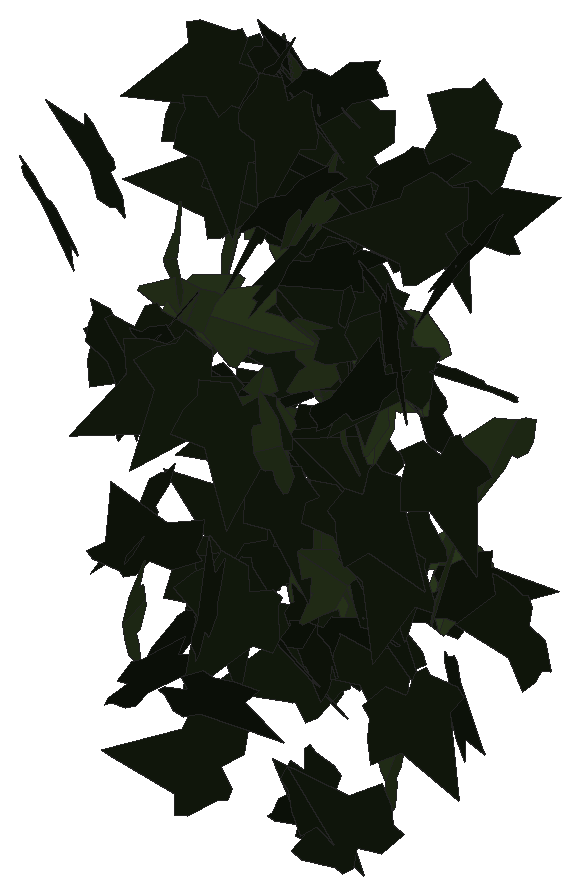
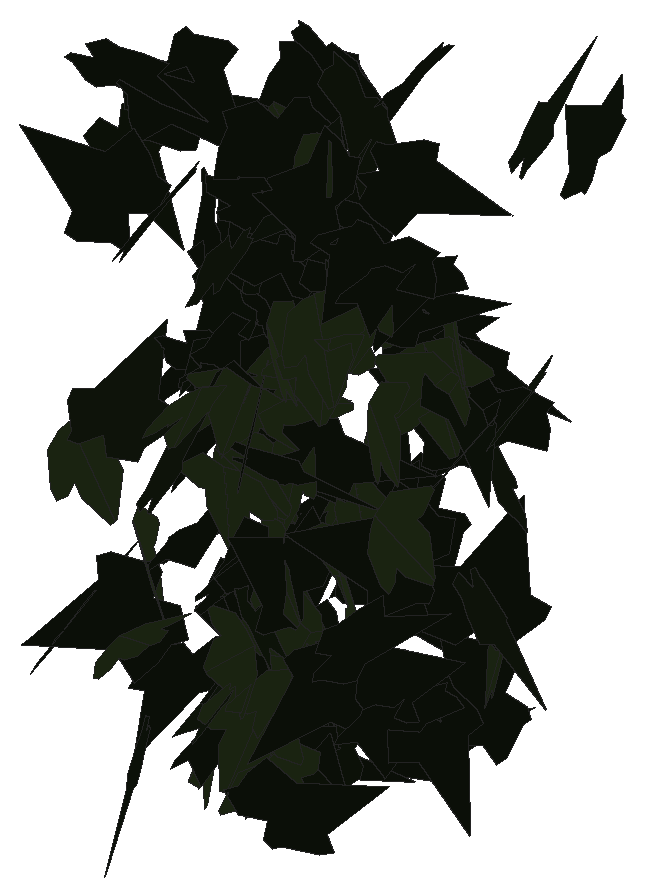
# SketchUp Ruby script. Lengths in inches.
U = 1.inch
M = Sketchup.active_model
def pt(a) = Geom::Point3d.new(a.map { |v| v * U })
def face(e, loops, mat)
  f = e.add_face(loops[0].map { |a| pt(a) })
  loops[1..].each { |l| e.add_face(l.map { |a| pt(a) }).erase! }
  f.material = f.back_material = mat if mat
  f
end
# faces: each face lists its corners as indices into pts; further lists are holes
def faces(e, pts, list, mat = nil) = list.each { |f| face(e, (f[0].is_a?(Array) ? f : [f]).map { |l| l.map { |i| pts[i] } }, mat) }
# xy, xz, yz: faces in a plane at the given z, y or x. An outline is a flat list of corners, or four numbers for a rectangle; further outlines are holes
def ring(l) = l.size == 4 ? [[l[0], l[1]], [l[2], l[1]], [l[2], l[3]], [l[0], l[3]]] : l.each_slice(2).to_a
def flat(e, list, mat, &to3) = list.each { |f| face(e, (f[0].is_a?(Array) ? f : [f]).map { |l| ring(l).map { |u, v| to3.(u, v) } }, mat) }
def xy(e, z, list, mat = nil) = flat(e, list, mat) { |x, y| [x, y, z] }
def xz(e, y, list, mat = nil) = flat(e, list, mat) { |x, z| [x, y, z] }
def yz(e, x, list, mat = nil) = flat(e, list, mat) { |y, z| [x, y, z] }
def lines(e, pts, list) = list.each { |a, b| e.add_line(pt(pts[a]), pt(pts[b])) }
# prism: a flat outline (further loops are holes) pulled along v
def prism(e, loops, v, mat = nil)
  f = face(e, loops, mat); d = Geom::Vector3d.new(v.map { |x| x * U })
  f.pushpull(f.normal.samedirection?(d) ? d.length : -d.length)
end
def box(e, o, s, mat = nil) = prism(e, [[o, [o[0] + s[0], o[1], o[2]], [o[0] + s[0], o[1] + s[1], o[2]], [o[0], o[1] + s[1], o[2]]]], [0, 0, s[2]], mat)
def at(x, y, z, deg = 0) = Geom::Transformation.translation(pt([x, y, z])) * Geom::Transformation.rotation(ORIGIN, Z_AXIS, deg.degrees)
def axes(o, x, y, z) = Geom::Transformation.new([*x, 0, *y, 0, *z, 0, *pt(o).to_a, 1])
def part(name) = M.definitions.add(name)
# library, detail: a bought-in or finely detailed component or shape, given as its bounding box
def library(name, o, s) = part(name).tap { |d| box(d.entities, o, s) }
def detail(e, o, s) = box(e.add_group.entities, o, s)
def put(e, d, t, mat = nil) = e.add_instance(d, t).tap { |i| i.material = mat if mat }
def group(e, t, mat = nil) = e.add_group.tap { |g| g.transformation = t; g.material = mat if mat }.entities
root = M.entities
M.materials.add("efeu1").color = [18, 25, 13]
M.materials.add("efeu2").color = [43, 57, 29]
c1 = part("ivyleaf_9")
p = [[1.54,2.16,1.25],[1.36,2.04,1.19],[-0.21,0.99,0.68],[-0.71,1.11,0.82],[-0.85,0.86,0.67],[-0.8,0.17,0.21],
  [-0.9,-0.01,0.1],[-0.67,-0.16,-0.02],[-0.08,-0.08,-0.05],[-0.03,-0.6,-0.4],[0.65,-0.88,-0.66],[0.83,-0.6,-0.49],
  [1.29,-0.42,-0.43],[1.8125,-0.07,-0.26],[1.21,0.44,0.15]]
faces(c1.entities,p,[[0,1,2,3,4,5,6,7,8,9,10,11,12,13,14]],"efeu1")
c2 = part("ivyleaf_10")
p = [[0,0.5,-0.03],[-0.0625,2.02,-0.43],[-0.19,2.01,-0.46],[-0.54,1.05,-0.29],[-0.52,0.625,-0.18],[-0.83,0.76,-0.28],
  [-1.16,0.64,-0.33],[-1.15,0.33,-0.24],[-0.77,-0.39,0.02],[-0.3,-0.51,0.16],[0.04,-0.48,0.23],[-0.02,2.01,-0.4375],
  [-0.06,2.01,-0.43],[0.04,-0.49,0.23],[0.67,-0.49,0.14],[1.38,0.36,-0.2],[1.375,0.51,-0.24],[0.81,0.65,-0.19],
  [0.62,0.59,-0.15],[0.6,1.09,-0.28],[0.5,1.23,-0.31]]
faces(c2.entities,p,[[0,1,2,3,4,5,6,7,8,9,10],[11,12,0,13,14,15,16,17,18,19,20]],"efeu2")
put(root,c1,axes([47.28,216.89,235.39],[0.45431,0.18289,0.10075],[0.09275,0.0394,-0.48974],[-0.18708,0.46368,0.00187]))
put(root,c1,axes([44.5625,217.46,241],[0.14292,-0.31641,0.35981],[0.16736,-0.31886,-0.34687],[0.44896,0.21958,0.01477]))
put(root,c1,axes([49.17,217.66,233.6],[0.12864,0.03086,0.48218],[-0.4817,0.0471,0.12549],[-0.03767,-0.49682,0.04185]))
put(root,c1,axes([48.48,217.62,234.32],[0.29957,-0.33555,-0.21831],[-0.12796,0.17811,-0.44934],[0.37932,0.32509,0.02084]))
put(root,c1,axes([47.18,217.97,238.78],[-0.20004,-0.4453,-0.10814],[0.0408,0.10022,-0.48815],[0.45642,-0.20412,-0.00376]))
put(root,c2,axes([47.98,217.66,238.68],[-0.22897,0.0956,0.43409],[-0.43182,0.06792,-0.24273],[-0.10538,-0.48605,0.05146]))
put(root,c1,axes([48.26,217.8125,233.48],[0.39361,0.26764,-0.15311],[0.12772,0.08446,0.47598],[0.28064,-0.41381,-0.00188]))
put(root,c1,axes([44.93,218.18,241.22],[0.19498,-0.45249,0.08506],[-0.02724,0.08087,0.49266],[-0.45961,-0.19675,0.00689]))
put(root,c1,axes([46.44,218.41,233.39],[-0.1512,-0.06618,0.47197],[-0.43354,-0.18655,-0.16504],[0.19794,-0.45915,-0.00097]))
put(root,c1,axes([45.84,218.32,238.45],[-0.46631,-0.01893,0.17942],[-0.17944,-0.00299,-0.46668],[0.01874,-0.49963,-0.004]))
put(root,c1,axes([46.72,217.84,235.67],[-0.01158,0.13161,0.48223],[-0.0926,0.47344,-0.13144],[-0.49121,-0.09236,0.01341]))
put(root,c1,axes([46.23,218.48,238.66],[-0.36119,-0.32993,0.10337],[-0.0728,-0.07356,-0.48917],[0.33799,-0.36842,0.0051]))
put(root,c1,axes([45.38,218.1,234.3125],[0.24314,0.25187,0.35699],[0.1949,0.30312,-0.3466],[-0.39102,0.3077,0.04922]))
put(root,c2,axes([45.29,218.2,235.1],[-0.03687,0.11331,0.4856],[-0.32453,0.36423,-0.10963],[-0.37858,-0.32326,0.04669]))
put(root,c1,axes([46.55,218.84,235.6],[-0.43672,-0.23988,-0.04162],[0.04043,0.01284,-0.4982],[0.24008,-0.43851,0.00818]))
put(root,c1,axes([48.26,218.67,238.86],[0.26417,0.36513,0.21655],[-0.12708,-0.17534,0.45067],[0.40505,-0.29314,0.00017]))
put(root,c1,axes([45.07,218.82,235.625],[0.34526,0.08136,0.35238],[-0.34374,-0.07758,0.35471],[0.1124,-0.4872,0.00236]))
put(root,c1,axes([46.08,218.91,241.97],[0.08588,-0.49223,0.01838],[0.004,-0.01796,-0.49966],[0.49255,0.08597,0.00085]))
put(root,c1,axes([44.52,218.97,238.44],[0.13607,-0.45073,0.16832],[0.05399,-0.15951,-0.47079],[0.47809,0.14629,0.00526]))
put(root,c1,axes([47.38,218.61,241.54],[0.04432,0.49482,-0.05648],[-0.00697,-0.05609,-0.4968],[-0.49798,0.04482,0.00192]))
put(root,c1,axes([45.79,219.24,236.79],[-0.06497,0.02785,0.49498],[0.09982,-0.48825,0.04057],[0.48561,0.10409,0.05788]))
put(root,c1,axes([44.76,218.95,238.59],[-0.14023,-0.24982,-0.40979],[0.20978,0.35208,-0.28642],[0.43166,-0.25225,0.00607]))
put(root,c2,axes([46.35,218.83,239.37],[-0.16308,-0.05724,-0.46918],[0.44267,0.15546,-0.17284],[0.16566,-0.47176,-0.00003]))
put(root,c1,axes([45.08,219.05,238.15],[0.20355,-0.10053,0.44549],[0.38513,-0.22435,-0.2266],[0.24545,0.43539,-0.0139]))
put(root,c1,axes([44.67,218.84,237.48],[-0.1833,0.43318,0.16957],[0.06858,-0.15511,0.47036],[0.46011,0.19569,-0.00255]))
put(root,c1,axes([47.17,218.85,240.39],[-0.24952,0.42755,0.07031],[-0.04339,0.05606,-0.49495],[-0.43111,-0.2531,0.00913]))
put(root,c1,axes([44.92,219.07,236.14],[-0.37205,0.32559,-0.07466],[0.04941,-0.05689,-0.49429],[-0.33036,-0.37518,0.01016]))
put(root,c1,axes([46.82,219.28,242.3],[-0.39904,-0.10547,-0.28221],[0.28159,0.03596,-0.4116],[0.10712,-0.48743,0.0307]))
put(root,c1,axes([48.28,219.01,237.48],[0.16164,-0.32661,-0.34234],[-0.12106,0.32117,-0.36358],[0.4574,0.20043,0.02475]))
put(root,c1,axes([45.14,219.03,238.71],[-0.14312,0.47706,0.04391],[-0.01783,0.04049,-0.49804],[-0.47875,-0.14412,0.00542]))
put(root,c2,axes([47.08,219.26,240.7],[0.0867,-0.46732,0.15521],[-0.00098,0.15743,0.47457],[-0.49242,-0.0826,0.02638]))
put(root,c1,axes([48.18,219.55,239.8],[-0.07664,0.01559,-0.49385],[0.49045,-0.05814,-0.07795],[-0.05986,-0.49636,-0.00638]))
put(root,c2,axes([45.23,219.17,239.67],[-0.14352,0.19169,0.43893],[-0.39852,0.20637,-0.22043],[-0.26568,-0.41312,0.09355]))
put(root,c1,axes([45.77,219.5,235.29],[-0.29498,-0.12088,-0.38519],[0.36396,0.1268,-0.31852],[0.17469,-0.4683,0.01319]))
put(root,c1,axes([44.86,219.75,237.9],[-0.01501,-0.42492,0.2631],[0.03157,-0.2635,-0.42376],[0.49878,0.00389,0.03474]))
put(root,c1,axes([46.55,219.55,236.81],[0.13412,-0.47881,-0.05246],[-0.01272,0.05091,-0.49724],[0.48151,0.13471,0.00148]))
put(root,c1,axes([45.35,219.35,234.72],[-0.13131,0.44988,-0.17426],[0.05746,-0.16473,-0.46858],[-0.47902,-0.14309,-0.00844]))
put(root,c2,axes([45.29,219.46,238.99],[-0.39842,-0.2409,0.18229],[-0.16363,-0.08153,-0.46538],[0.25394,-0.43049,-0.01387]))
put(root,c1,axes([48.1,219.8125,236.21],[-0.06572,-0.47098,0.15445],[0.0166,-0.15781,-0.47415],[0.49538,-0.05719,0.03638]))
put(root,c2,axes([47.24,219.82,235.625],[-0.11689,-0.31436,-0.37083],[-0.13415,-0.34573,0.33537],[-0.46727,0.17789,-0.00352]))
put(root,c1,axes([48.8,219.79,241.01],[-0.25162,-0.04846,0.42935],[-0.41317,-0.11837,-0.2555],[0.1264,-0.48336,0.01952]))
put(root,c1,axes([48.51,219.875,241.77],[-0.03218,0.25489,-0.42895],[0.0043,-0.42968,-0.25565],[-0.49894,-0.02014,0.02546]))
put(root,c2,axes([45.16,219.51,238.84],[0.20781,0.24836,0.38096],[0.16667,0.34811,-0.31786],[-0.42312,0.2591,0.06189]))
put(root,c1,axes([48.37,219.71,234.41],[0.05073,-0.35653,-0.34686],[-0.06275,0.34129,-0.35998],[0.49345,0.08006,-0.01012]))
put(root,c2,axes([45.95,219.93,237.32],[0.37256,-0.04324,0.33065],[0.32776,-0.04387,-0.37504],[0.06144,0.49619,-0.00434]))
put(root,c1,axes([48.71,219.93,237.75],[0.10704,-0.45706,-0.17216],[-0.0305,0.16965,-0.46935],[0.48745,0.11098,0.00844]))
put(root,c1,axes([46.1,219.55,242.04],[-0.0474,0.41223,0.27896],[-0.068,0.27223,-0.41384],[-0.49308,-0.07717,0.03025]))
put(root,c1,axes([46.01,220.09,240.3125],[-0.35612,0.16064,-0.31204],[0.24615,-0.20256,-0.3852],[-0.25017,-0.42798,0.06518]))
put(root,c2,axes([48.13,219.59,233.42],[0.04917,0.0415,-0.49584],[-0.09062,0.49067,0.03208],[0.48926,0.08671,0.05578]))
put(root,c1,axes([45.21,220.12,235.06],[-0.08371,-0.46865,-0.15283],[0.02785,0.15028,-0.47607],[0.49216,-0.08821,0.00094]))
put(root,c1,axes([49.08,220.02,240.79],[-0.24626,0.37324,-0.22371],[0.09564,-0.20434,-0.4462],[-0.42451,-0.26256,0.02925]))
put(root,c1,axes([47.87,220.21,236.47],[0.01179,-0.49983,-0.00529],[-0.00055,0.00527,-0.49997],[0.49986,0.0118,-0.00042]))
put(root,c1,axes([45.89,220.06,234.32],[0.41009,-0.23058,0.16928],[0.14697,-0.084,-0.47047],[0.2454,0.43563,-0.00112]))
put(root,c1,axes([46.64,220.26,234.1],[-0.39418,-0.07273,0.29889],[-0.28828,-0.08215,-0.40018],[0.10732,-0.48781,0.02283]))
put(root,c1,axes([46.68,220.23,240.08],[0.27394,0.07053,0.41229],[-0.39656,-0.11294,0.28281],[0.13302,-0.48194,-0.00594]))
put(root,c1,axes([46.74,219.94,234.65],[0.01144,0.07242,-0.4946],[-0.49028,-0.09482,-0.02522],[-0.09745,0.48556,0.06884]))
put(root,c2,axes([46.81,220.34,238.3],[-0.24042,-0.28924,-0.32946],[-0.19061,-0.26941,0.37561],[-0.3948,0.3062,0.01928]))
put(root,c1,axes([46.83,219.82,239.89],[0.31862,0.38518,-0.01098],[-0.00702,-0.00844,-0.49988],[-0.38527,0.31869,0.00003]))
put(root,c1,axes([45.17,220.35,241.83],[-0.05424,-0.10856,-0.48505],[-0.22862,-0.4278,0.12131],[-0.44135,0.23495,-0.00323]))
put(root,c2,axes([45.55,220.21,236.93],[-0.30103,-0.39797,0.03171],[0.02108,0.02382,0.49899],[-0.39867,0.30175,0.00244]))
put(root,c1,axes([46.95,220.41,236.26],[0.03706,-0.48761,0.10425],[0.16934,-0.08601,-0.46252],[0.46899,0.06958,0.15877]))
put(root,c1,axes([47.79,220.41,238.78],[-0.47491,-0.15614,0.00898],[-0.00833,-0.00341,-0.49992],[0.15618,-0.47498,0.00064]))
put(root,c1,axes([45.23,220.45,240.125],[-0.2596,-0.0531,0.42402],[-0.40942,-0.11121,-0.26459],[0.12241,-0.48457,0.01426]))
put(root,c1,axes([45.66,220.32,240.59],[0.09528,-0.11327,0.47759],[0.40337,-0.25914,-0.14193],[0.27967,0.41233,0.04199]))
put(root,c1,axes([46.84,220.02,234.71],[0.34633,0.33769,-0.12659],[-0.09636,-0.08249,-0.48364],[-0.34753,0.35939,0.00794]))
put(root,c2,axes([45.7,220.24,236.07],[0.36658,-0.33997,0.00618],[-0.00391,0.00488,0.49996],[-0.34001,-0.3666,0.00092]))
put(root,c1,axes([45.57,220.25,235.38],[-0.0687,0.05447,0.49225],[-0.46083,0.17502,-0.08368],[-0.18143,-0.46519,0.02615]))
put(root,c1,axes([47.11,220.48,238.83],[-0.09748,0.09989,0.48012],[-0.45958,-0.18942,-0.0539],[0.17112,-0.45182,0.12875]))
put(root,c2,axes([46.63,220.27,235.84],[-0.48536,0.01008,0.11969],[-0.11978,-0.00317,-0.48543],[-0.00902,-0.49989,0.0055]))
put(root,c2,axes([48.41,220.47,236.18],[0.28858,-0.40412,0.05839],[0.03401,-0.04746,-0.49658],[0.4069,0.29058,0.00009]))
put(root,c1,axes([46.11,220.45,240.57],[-0.39925,0.08176,0.28968],[-0.28237,0.06491,-0.4075],[-0.10424,-0.48898,-0.00566]))
put(root,c1,axes([44.85,220.2,237.04],[0.22329,-0.01501,0.44712],[0.44279,0.07876,-0.21848],[-0.06387,0.49353,0.04847]))
put(root,c1,axes([47.26,220.25,239.73],[0.45456,-0.04872,-0.20249],[-0.20072,0.02727,-0.45713],[0.05558,0.49687,0.00523]))
put(root,c2,axes([46.34,220.4,235.85],[0.22532,-0.02651,-0.44557],[0.4425,-0.05216,0.22687],[-0.05851,-0.49656,-0.00004]))
put(root,c1,axes([48.86,220.66,242.07],[-0.47429,-0.11771,0.1058],[-0.09906,-0.03991,-0.48846],[0.12343,-0.48431,0.01454]))
put(root,c1,axes([46.02,220.67,238.22],[-0.17949,-0.19147,-0.42558],[-0.27807,-0.32231,0.26228],[-0.37478,0.33084,0.00923]))
put(root,c1,axes([47.17,220.61,234.44],[0.06722,-0.48369,-0.10734],[-0.02134,0.10539,-0.4883],[0.495,0.07023,-0.00648]))
put(root,c1,axes([45.52,220.88,241.44],[0.03168,-0.3476,0.35801],[0.05938,-0.35356,-0.34853],[0.49545,0.0646,0.01887]))
put(root,c1,axes([46.99,220.66,238.71],[-0.31634,-0.27659,-0.27097],[0.2159,0.16446,-0.41993],[0.32142,-0.38269,0.01538]))
put(root,c1,axes([46.79,220.45,239.42],[-0.26379,-0.0344,-0.42336],[-0.41991,-0.0539,0.26603],[-0.06394,0.49589,-0.00045]))
put(root,c1,axes([46.6,220.86,236.51],[0.00612,0.0465,0.4978],[-0.35879,-0.34629,0.03676],[0.34818,-0.35766,0.02913]))
put(root,c1,axes([47.09,220.875,240.09],[0.29268,-0.39355,-0.09727],[0.06131,-0.07561,0.49043],[-0.40073,-0.299,0.004]))
put(root,c1,axes([46.52,220.51,242.02],[0.08891,0.41605,-0.26268],[-0.039,-0.26013,-0.42522],[-0.49048,0.0961,-0.01381]))
put(root,c1,axes([46.93,220.6,238.25],[-0.07681,0.07763,0.48793],[-0.47472,0.12524,-0.09466],[-0.13691,-0.4778,0.05447]))
put(root,c1,axes([45.79,220.28,235.45],[0.02004,-0.07159,-0.49444],[-0.07123,0.48938,-0.07375],[0.4945,0.07339,0.00941]))
put(root,c1,axes([45.84,220.55,241.7],[0.44324,-0.22903,-0.03287],[-0.03002,0.01351,-0.49891],[0.22942,0.44425,-0.00177]))
put(root,c2,axes([46.47,220.66,238.68],[0.13214,0.04788,0.47984],[-0.45082,-0.16434,0.14055],[0.17117,-0.46979,-0.00026]))
put(root,c2,axes([45.27,220.52,240.46],[-0.46951,0.17192,-0.00199],[0.001,-0.00308,-0.49999],[-0.17193,-0.4695,0.00255]))
put(root,c1,axes([47.01,220.7,235.02],[0.31221,-0.39035,-0.0123],[-0.00248,0.01377,-0.4998],[0.39054,0.31215,0.00667]))
put(root,c2,axes([46.42,220.74,234.14],[0.24995,0.38941,-0.18943],[-0.09505,-0.16406,-0.46266],[-0.42248,0.26729,-0.00799]))
put(root,c1,axes([46.9,220.76,240.99],[-0.34017,0.06273,0.36104],[-0.36386,0.00058,-0.34293],[-0.04344,-0.49605,0.04525]))
put(root,c2,axes([46.23,220.57,238.1],[-0.44929,0.21548,0.04128],[-0.03744,0.01739,-0.49829],[-0.21618,-0.45085,0.00051]))
put(root,c2,axes([47.04,220.61,237.71],[0.17713,-0.04371,-0.46553],[-0.43163,0.17612,-0.18077],[0.17978,0.46591,0.02466]))
put(root,c1,axes([46.68,220.9,236.34],[-0.3545,0.09764,-0.33881],[0.30148,-0.16522,-0.36306],[-0.18285,-0.4617,0.05827]))
put(root,c2,axes([46.28,220.65,235.24],[0.16575,0.46831,0.05664],[0.01445,0.05497,-0.49676],[-0.47151,0.16631,0.00469]))
put(root,c2,axes([46.78,220.72,238.65],[0.43448,0.14969,0.19703],[0.18719,0.06154,-0.45954],[-0.16183,0.47308,-0.00257]))
put(root,c1,axes([44.55,220.83,240.98],[-0.08274,-0.43421,-0.23371],[0.06371,0.22557,-0.44165],[0.48897,-0.10287,0.018]))
put(root,c1,axes([49.06,221.12,235.05],[0.20247,-0.39494,-0.23029],[0.10411,-0.20541,0.44381],[-0.44516,-0.22767,-0.00094]))
put(root,c1,axes([46.33,220.85,233.64],[-0.08164,0.05045,0.4907],[-0.49147,0.03442,-0.08531],[-0.04239,-0.49626,0.04397]))
put(root,c1,axes([47.86,220.875,240.7],[0.19255,-0.45908,-0.04659],[-0.01274,0.04518,-0.49779],[0.46126,0.19289,0.0057]))
put(root,c2,axes([44.55,221.04,237.92],[0.04184,-0.39803,0.2997],[0.04178,-0.2969,-0.40013],[0.49649,0.05853,0.00842]))
put(root,c1,axes([46.93,221.08,236.375],[0.02828,-0.48033,-0.13597],[0.00628,-0.13583,0.48115],[-0.49916,-0.02892,-0.00165]))
put(root,c2,axes([45.85,220.67,241.9],[-0.41021,0.24973,0.13916],[-0.12865,0.05611,-0.4799],[-0.2553,-0.42952,0.01822]))
put(root,c2,axes([46.71,220.9375,235.625],[-0.28568,0.16995,-0.3735],[0.28698,-0.24256,-0.32986],[-0.29331,-0.40284,0.04104]))
put(root,c2,axes([47.25,221.01,238.53],[-0.23481,-0.44122,0.01381],[0.32178,-0.18178,-0.33677],[0.3022,-0.14926,0.36932]))
put(root,c2,axes([46.55,220.84,234.87],[-0.47827,-0.0779,-0.12326],[0.1238,0.0064,-0.48439],[0.07704,-0.49385,0.01316]))
put(root,c2,axes([46.53,220.75,236.86],[-0.19708,0.03984,0.45779],[-0.44544,0.10582,-0.20097],[-0.1129,-0.48705,-0.00622]))
put(root,c1,axes([48.28,220.5625,235.54],[0.02553,0.18907,-0.46217],[0.04865,0.45963,0.19072],[0.49697,-0.05471,0.00507]))
put(root,c2,axes([44.63,221.13,239.29],[0.15512,-0.43009,0.20239],[0.12874,-0.16693,-0.45339],[0.45756,0.19278,0.05895]))
put(root,c1,axes([45.0625,221.32,236.34],[-0.20331,-0.19218,0.4144],[-0.28107,-0.30493,-0.27931],[0.36009,-0.34653,0.01596]))
put(root,c1,axes([46.35,221.11,238.18],[-0.44803,0.06809,0.21126],[-0.22046,-0.08127,-0.44135],[-0.02577,-0.48863,0.10284]))
put(root,c2,axes([46.8125,221,237.72],[0.49133,0.04181,0.08273],[0.08287,0.00179,-0.49308],[-0.04153,0.49825,-0.00517]))
put(root,c1,axes([45.35,221.0625,241.68],[0.31904,-0.22469,0.31262],[0.24812,-0.19043,-0.39009],[0.29436,0.40404,-0.01001]))
put(root,c1,axes([48.3,220.95,240.55],[0.0548,-0.05132,0.49433],[0.46906,-0.15902,-0.06851],[0.16425,0.47125,0.03072]))
put(root,c2,axes([47.93,221.33,235.48],[-0.30011,-0.27625,0.28916],[0.21351,-0.41638,-0.17619],[0.33815,0.01772,0.36789]))
put(root,c1,axes([48.21,221.36,238.02],[-0.38765,-0.22282,0.22378],[0.21967,-0.44481,-0.06238],[0.22688,0.04995,0.44275]))
put(root,c1,axes([46.25,221.27,238.78],[0.06521,-0.0169,-0.49544],[0.44677,-0.21453,0.06612],[-0.21481,-0.45132,-0.01287]))
put(root,c2,axes([45.47,220.97,239.76],[0.2878,0.40826,0.02229],[0.01305,0.01807,-0.4995],[-0.40866,0.2881,-0.00025]))
put(root,c2,axes([45.5,221.07,240.23],[-0.15383,-0.47446,0.03495],[-0.01076,-0.03325,-0.49878],[0.47563,-0.1542,0.00002]))
put(root,c2,axes([48.73,221.17,237.59],[-0.11776,-0.45791,0.16264],[-0.04893,-0.15532,-0.47274],[0.48347,-0.12725,-0.00823]))
put(root,c2,axes([45.98,221.21,239.85],[0.24645,-0.38977,0.19324],[0.12309,-0.15054,-0.46064],[0.41727,0.27461,0.02175]))
put(root,c1,axes([47.6,221.26,237.45],[0.19236,-0.45943,0.04386],[-0.00882,0.04384,0.498],[-0.46143,-0.19237,0.00876]))
put(root,c1,axes([46.02,220.75,236.55],[0.00045,-0.11288,0.48709],[0.30873,0.38321,0.08852],[-0.3933,0.30067,0.07005]))
put(root,c1,axes([44.68,221.02,241.38],[-0.12632,-0.26784,-0.40287],[0.21117,0.34409,-0.29498],[0.43526,-0.24467,0.02619]))
put(root,c1,axes([48.09,220.9,233.95],[0.28459,-0.12551,-0.39148],[-0.35568,0.16358,-0.31102],[0.20615,0.45551,0.00382]))
